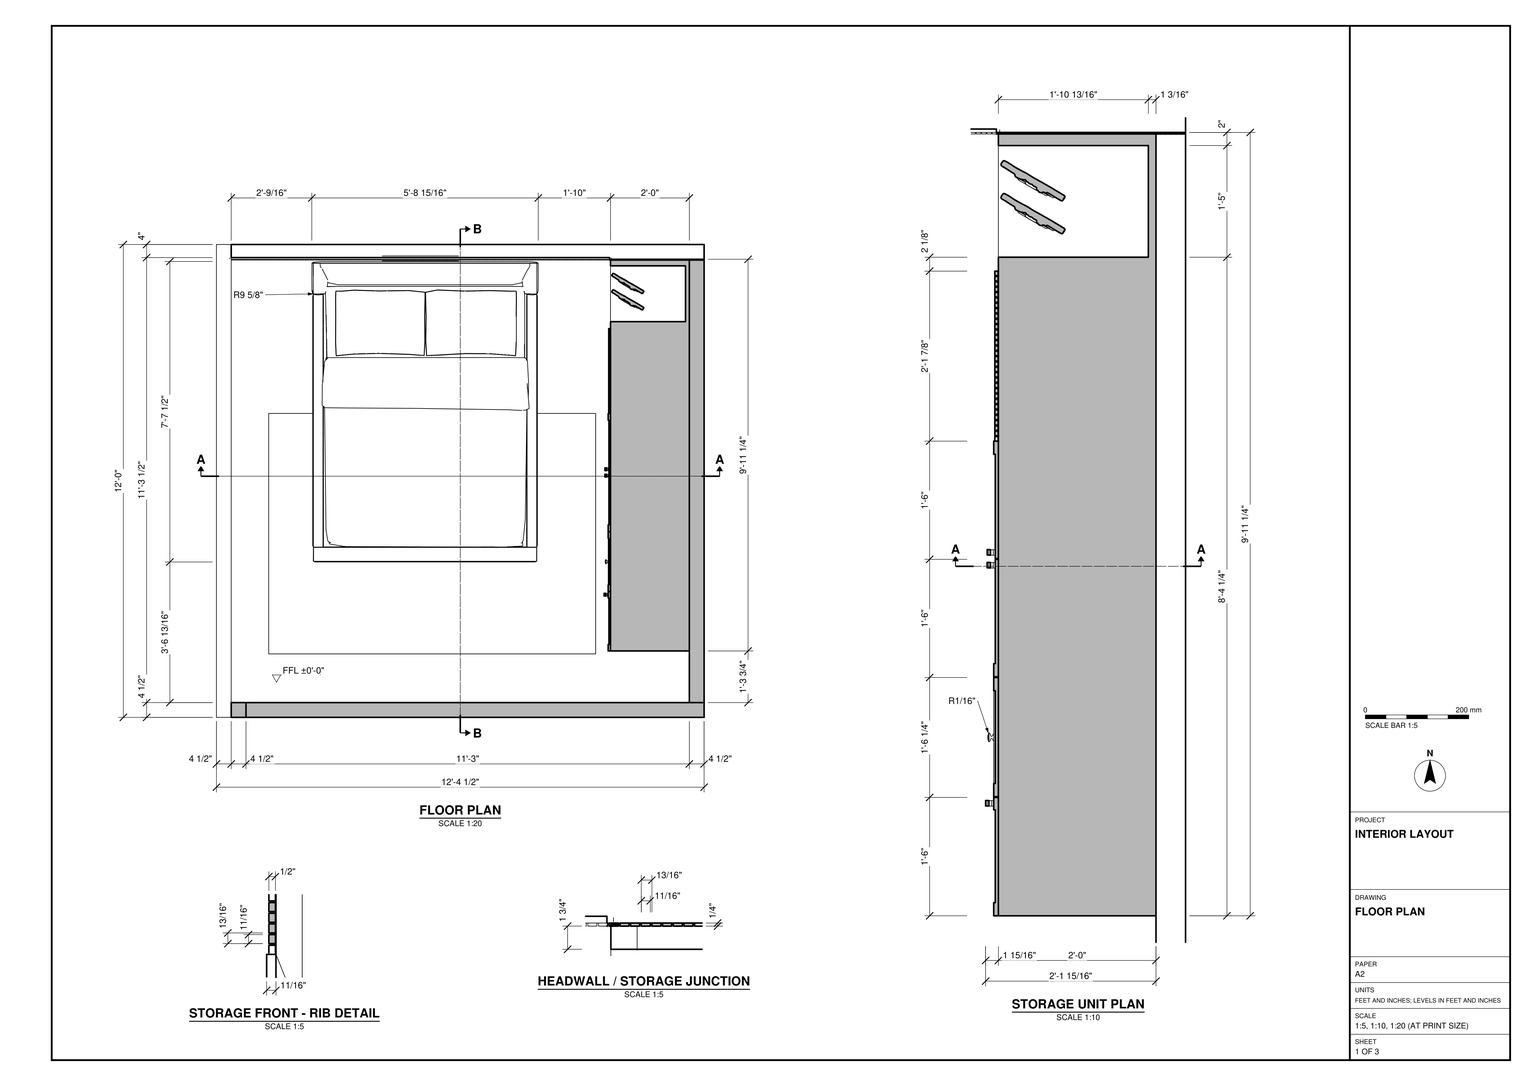
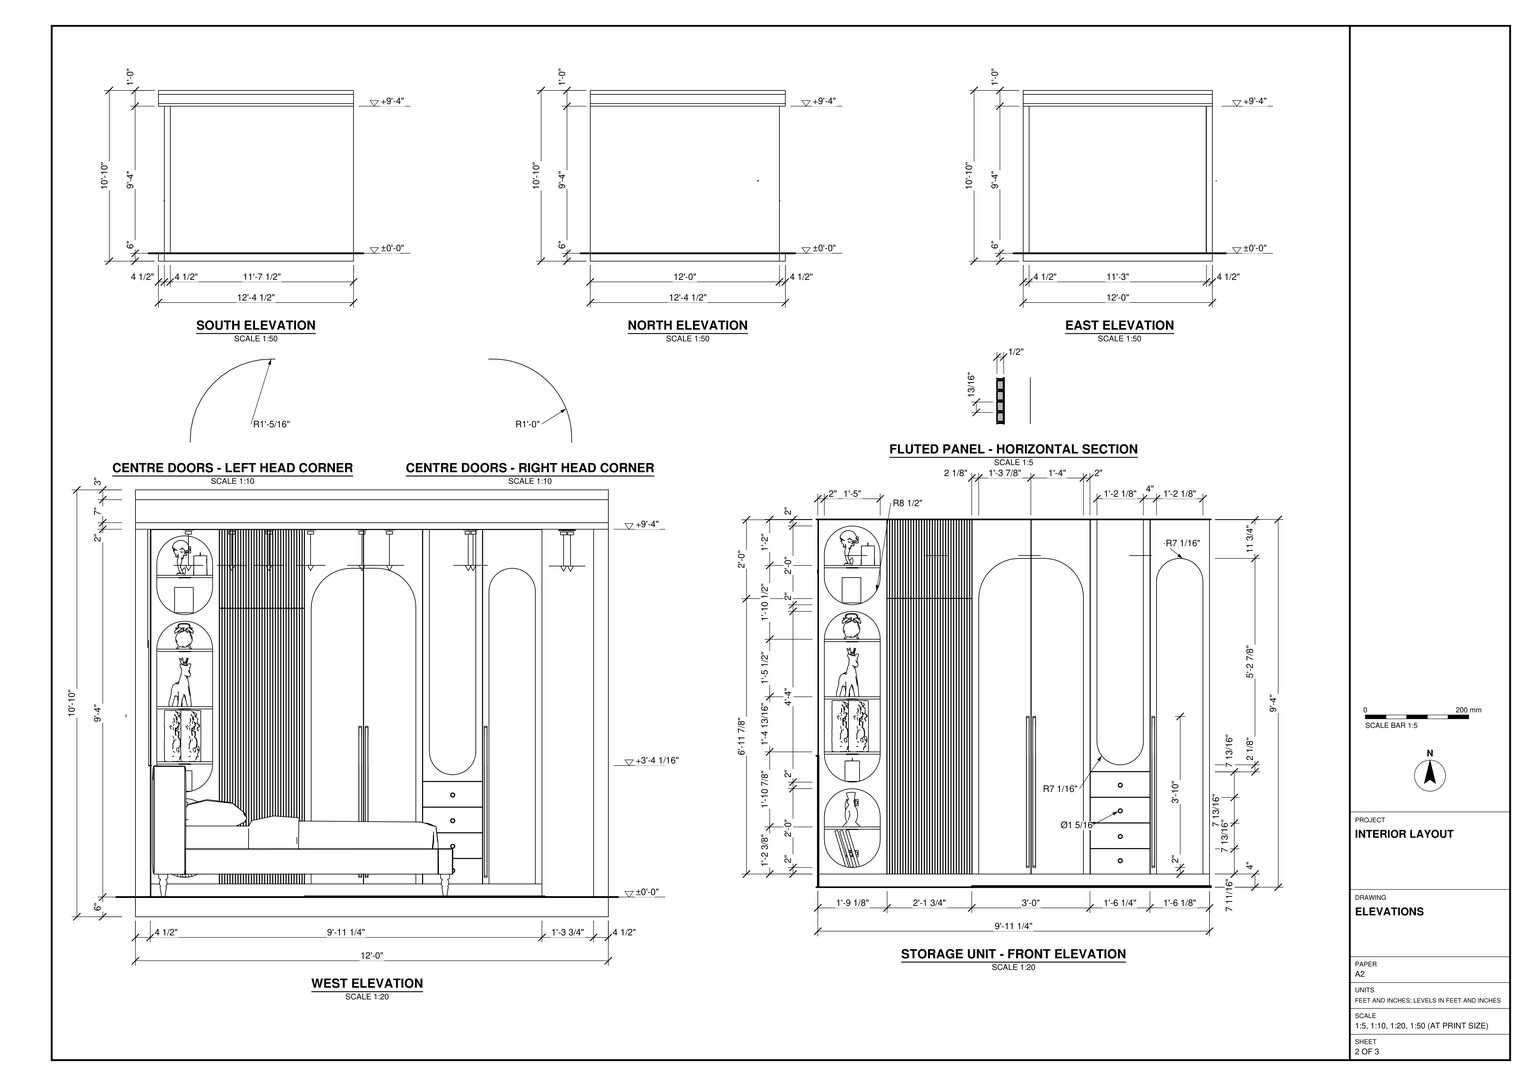
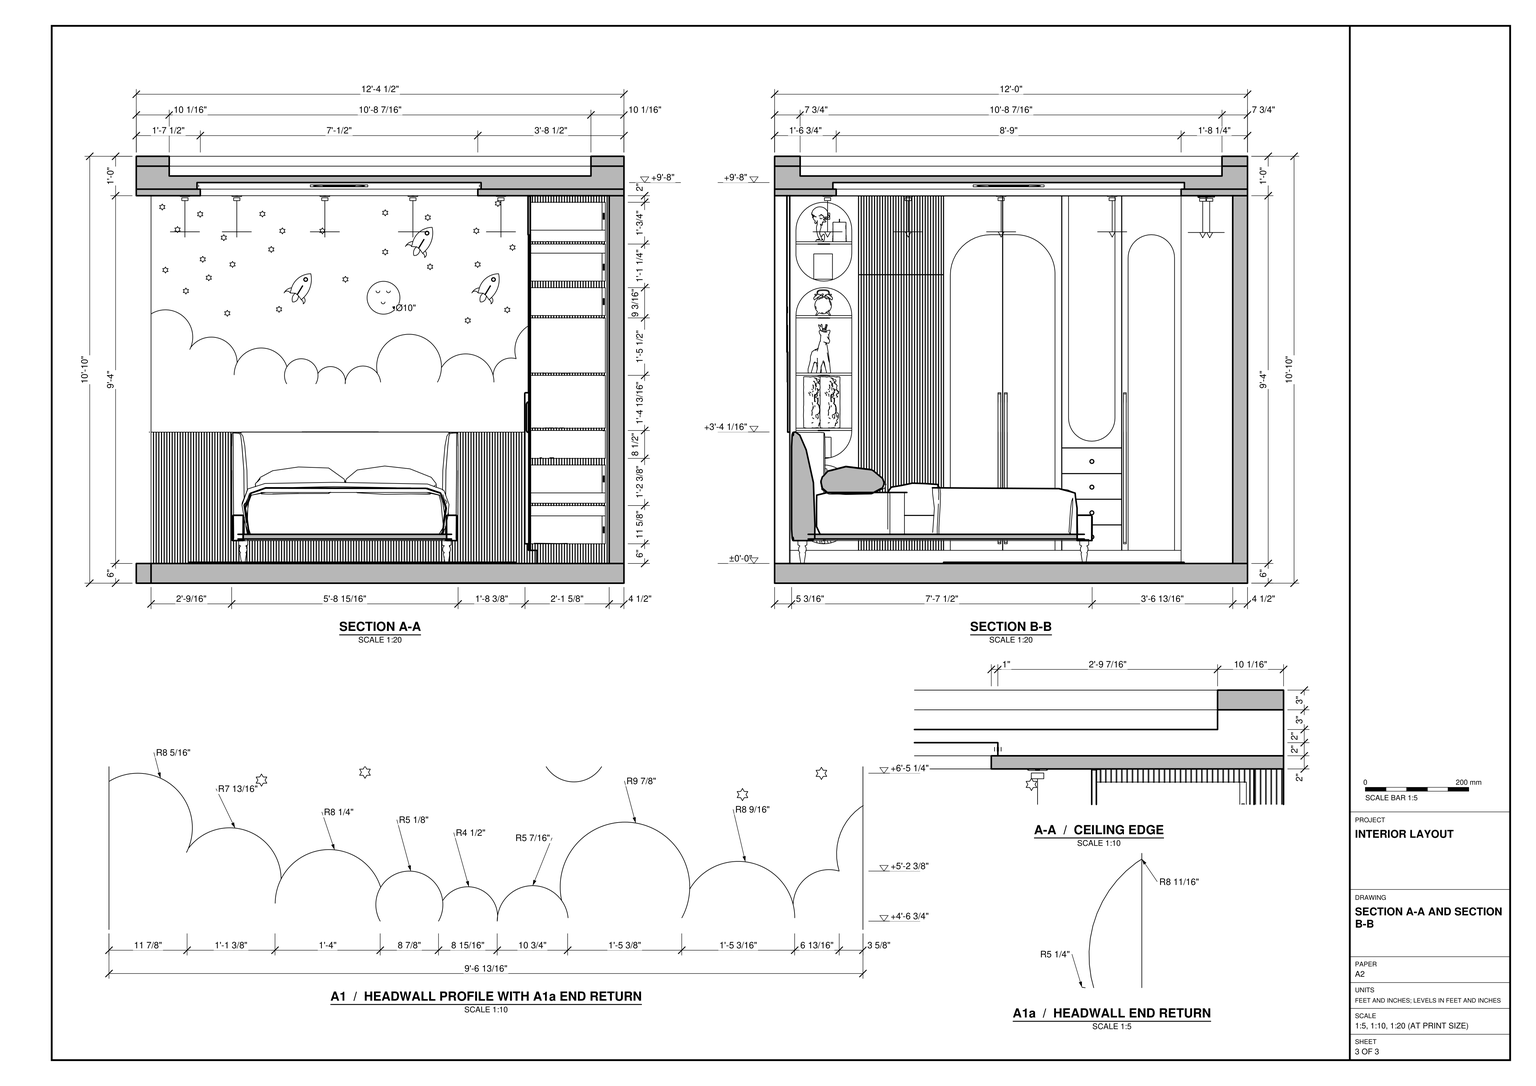
Build the bedroom interior in SketchUp from task_files/diagram_01.pdf. Work in feet and inches. Set the finished floor at ±0'-0" and make the overall model 12'-4 1/2" along X, 12'-2 7/8" along Y and 10'-10" high. Use the floor plan for placement and the sections for the floor slab, wall thicknesses and returns, clear height and stepped ceiling edge.

Place the bed with its head against the north wall and its foot facing the open floor area. Match the bed frame, raised headboard and footprint in plan and section. Behind the bed, model the ribbed lower panel and the scalloped headwall profile, including its curved end return. Fit the storage unit along the east wall with its fronts facing the bed. Follow the front elevation for the sequence of rounded display openings with shelves, a fluted bay, paired centre doors, a drawer stack and a tall end door. Use the enlarged details for the ribs and the junction with the headwall.

Decor and loose items, including the rug, shelf objects, wall decorations and lights, may be any suitable library components placed as shown. Keep the shell elements and each furniture or joinery piece in separate groups or components, and use components for repeated parts. Save one SketchUp model as output_files/bedroom_with_a_scalloped_headwall_and_fitted_storage.skp.

# SketchUp Ruby script. Lengths in inches.
U = 1.inch
M = Sketchup.active_model
def pt(a) = Geom::Point3d.new(a.map { |v| v * U })
def face(e, loops, mat)
  f = e.add_face(loops[0].map { |a| pt(a) })
  loops[1..].each { |l| e.add_face(l.map { |a| pt(a) }).erase! }
  f.material = f.back_material = mat if mat
  f
end
# faces: each face lists its corners as indices into pts; further lists are holes
def faces(e, pts, list, mat = nil) = list.each { |f| face(e, (f[0].is_a?(Array) ? f : [f]).map { |l| l.map { |i| pts[i] } }, mat) }
# xy, xz, yz: faces in a plane at the given z, y or x. An outline is a flat list of corners, or four numbers for a rectangle; further outlines are holes
def ring(l) = l.size == 4 ? [[l[0], l[1]], [l[2], l[1]], [l[2], l[3]], [l[0], l[3]]] : l.each_slice(2).to_a
def flat(e, list, mat, &to3) = list.each { |f| face(e, (f[0].is_a?(Array) ? f : [f]).map { |l| ring(l).map { |u, v| to3.(u, v) } }, mat) }
def xy(e, z, list, mat = nil) = flat(e, list, mat) { |x, y| [x, y, z] }
def xz(e, y, list, mat = nil) = flat(e, list, mat) { |x, z| [x, y, z] }
def yz(e, x, list, mat = nil) = flat(e, list, mat) { |y, z| [x, y, z] }
def lines(e, pts, list) = list.each { |a, b| e.add_line(pt(pts[a]), pt(pts[b])) }
# prism: a flat outline (further loops are holes) pulled along v
def prism(e, loops, v, mat = nil)
  f = face(e, loops, mat); d = Geom::Vector3d.new(v.map { |x| x * U })
  f.pushpull(f.normal.samedirection?(d) ? d.length : -d.length)
end
def box(e, o, s, mat = nil) = prism(e, [[o, [o[0] + s[0], o[1], o[2]], [o[0] + s[0], o[1] + s[1], o[2]], [o[0], o[1] + s[1], o[2]]]], [0, 0, s[2]], mat)
def at(x, y, z, deg = 0) = Geom::Transformation.translation(pt([x, y, z])) * Geom::Transformation.rotation(ORIGIN, Z_AXIS, deg.degrees)
def axes(o, x, y, z) = Geom::Transformation.new([*x, 0, *y, 0, *z, 0, *pt(o).to_a, 1])
def part(name) = M.definitions.add(name)
# library, detail: a bought-in or finely detailed component or shape, given as its bounding box
def library(name, o, s) = part(name).tap { |d| box(d.entities, o, s) }
def detail(e, o, s) = box(e.add_group.entities, o, s)
def put(e, d, t, mat = nil) = e.add_instance(d, t).tap { |i| i.material = mat if mat }
def group(e, t, mat = nil) = e.add_group.tap { |g| g.transformation = t; g.material = mat if mat }.entities
root = M.entities
M.materials.add("A08_Garnet_Shadow5").color = [28, 26, 30]
M.materials.add("DDR840RVS01100X").color = [126, 127, 125]
M.materials.add("Uniboard-L19-Putty-4K").color = [187, 181, 160]
c1 = part("Component\#11")
prism(c1.entities,[[[0.1875,0.74,0.15],[0.1875,0.74,16.59],[0.1875,0.74,16.61],[0.1875,0.73,16.625],[0.1875,0.73,16.64],[0.1875,0.72,16.66],[0.1875,0.71,16.67],[0.1875,0.7,16.68],[0.1875,0.6875,16.69],[0.1875,0.67,16.7],[0.1875,0.66,16.71],[0.1875,0.64,16.72],[0.1875,0.625,16.72],[0.1875,0.61,16.72],[0.18,0,16.72],[0.18,0,15.68],[0.18,0.14,15.68],[0.18,0.18,15.68],[0.18,0.22,15.67],[0.18,0.25,15.66],[0.18,0.29,15.64],[0.18,0.32,15.62],[0.18,0.35,15.59],[0.19,0.375,15.57],[0.1875,0.4,15.53],[0.1875,0.41,15.5],[0.1875,0.43,15.46],[0.1875,0.43,15.42],[0.1875,0.44,15.39],[0.1875,0.44,12.6],[0.1875,0.43,12.57],[0.1875,0.43,12.54],[0.1875,0.42,12.51],[0.1875,0.4,12.48],[0.19,0.38,12.45],[0.19,0.36,12.42],[0.18,0.34,12.4],[0.18,0.31,12.38],[0.18,0.28,12.37],[0.18,0.25,12.36],[0.18,0.22,12.35],[0.18,0.18,12.35],[0.18,0,12.35],[0.18,0,0],[0.1875,0.59,0],[0.1875,0.61,0],[0.1875,0.625,0.01],[0.1875,0.65,0.01],[0.1875,0.66,0.02],[0.1875,0.68,0.03],[0.1875,0.69,0.04],[0.1875,0.71,0.06],[0.1875,0.72,0.07],[0.1875,0.73,0.09],[0.1875,0.73,0.11],[0.1875,0.74,0.13]]],[-0.18,0,0],"A08_Garnet_Shadow5")
c2 = library("Interior Props 221 025",[-7.35,-1.5,-10.4],[14.7,1.56,20.81])
c3 = library("Decorative Deer 209 004",[-1.58,-4.16,0],[3.36,7.25,10.63])
c4 = library("Alarm Clock 114 007",[-2.86,-1.17,0.01],[5.71,2.99,7.86])
c5 = library("Interior Props 221 030",[-2.57,-3.63,-0.04],[5.13,7.27,11.89])
c6 = library("Decoration 111 063",[-2.51,-1.28,-0.03],[5.02,2.53,10.66])
c7 = library("Candle 111 040",[-2.11,-2.13,-0.02],[4.23,4.26,6.92])
c8 = library("Block 237 020",[-7.27,-8.35,0],[14.55,16.7,1.34])
c9 = part("Picture 288 039")
xz(c9.entities,-0.24,[[0.99,-15.21,-10.86,-15.18,-0.62,1.61],[0.99,-15.21,-0.62,1.61,10.87,-15.17],[0.67,-15.2,-0.25,2.42,-10.86,-15.16],[0.67,-15.2,10.89,1.32,-0.25,2.42],[0.67,-15.2,10.89,-15.1875,10.89,1.32],
  [-10.86,-15.18,-10.9,-1.29,-0.62,1.61],[10.87,-15.17,-0.62,1.61,10.9,-0.22],[-10.86,-15.16,-0.25,2.42,-10.89,2.08],[-10.9,-1.29,-10.9,15.22,-0.62,1.61],[10.9,-0.22,-0.62,1.61,10.88,15.2],
  [10.89,1.32,-1.31,15.2,-0.25,2.42],[10.89,1.32,10.89,15.21,-1.31,15.2],[-0.62,1.61,-10.9,15.22,-1.1,15.21],[-0.62,1.61,-1.1,15.21,10.88,15.2],[-10.89,2.08,-1.31,15.2,-10.9,15.2],
  [-10.89,2.08,-0.25,2.42,-1.31,15.2]])
xz(c9.entities,0,[[-12.08,-16.4,-12.1875,16.41,-11.52,3.74],[-12.08,-16.4,-11.45,-15.77,1.62,-15.8],[-12.08,-16.4,-11.52,3.74,-11.45,-15.77],[-12.08,-16.4,1.62,-15.8,11.44,-15.79],[-12.08,-16.4,11.44,-15.79,12.07,-16.375],
  [12.07,-16.375,11.44,-15.79,11.52,1.58],[12.07,-16.375,11.52,1.58,12.12,-2.15],[12.12,-2.15,11.52,1.58,12.07,16.36],[11.52,1.58,11.45,15.77,12.07,16.36],[-11.52,3.74,-12.1875,16.41,-11.43,15.75],
  [-11.43,15.75,-12.1875,16.41,-0.49,15.82],[11.45,15.77,-0.49,15.82,12.07,16.36],[-0.49,15.82,-12.1875,16.41,12.07,16.36]])
p = [[-12.19,-0.11,-1.23],[-12.2,-0.1,-16.51],[-11.65,-0.48,-4.41],[-11.48,-0.48,-15.9],[11.63,-0.48,-15.94],[12.2,-0.1,-16.52],
  [12.19,-0.11,-0.02],[-12.08,0,-16.4],[-12.12,-0.05,-16.53],[-12.21,-0.02,-16.4375],[-12.22,-0.0625,-3.89],[1.85,-0.0625,-16.53],
  [-0.625,-0.01,-16.52],[12.14,-0.02,-16.53],[12.21,-0.02,-16.43],[12.22,-0.0625,2.37],[12.07,0,-16.375],[-12.21,-0.01,0.01],
  [12.21,-0.01,16.52],[-12.1875,0,16.41],[12.12,0,-2.15],[-11.46,-0.47,-0.79],[-10.86,-0.24,-15.16],[-0.9,-0.47,-15.76],
  [0.67,-0.24,-15.2],[10.89,-0.24,-15.1875],[11.46,-0.47,1.83],[11.42,-0.47,15.71],[11.65,-0.48,15.96],[-11.45,0,-15.77],
  [-11.52,0,3.74],[-10.9,-0.24,-1.29],[-10.86,-0.24,-15.18],[1.62,0,-15.8],[0.99,-0.24,-15.21],[10.87,-0.24,-15.17],
  [11.44,0,-15.79],[10.9,-0.24,-0.22],[11.52,0,1.58],[-10.89,-0.24,2.08],[10.89,-0.24,1.32],[-12.2,-0.1,16.51],
  [-11.51,-0.48,15.89],[-12.22,-0.07,16.47],[12.07,0,16.36],[-10.9,-0.24,15.22],[-10.9,-0.24,15.2],[10.88,-0.24,15.2],
  [12.2,-0.1,16.51],[10.89,-0.24,15.21],[11.45,0,15.77],[12.22,-0.0625,16.53],[-11.43,0,15.75],[-1.71,-0.47,15.76],
  [-1.31,-0.24,15.2],[-0.49,0,15.82],[-1.1,-0.24,15.21],[-12.08,-0.01,16.52],[-1.82,-0.0625,16.53]]
faces(c9.entities,p,[[0,1,2],[1,3,2],[3,1,4],[1,5,4],[4,5,6],[7,8,9],[9,8,1],[1,0,10],
  [10,9,1],[8,11,1],[1,11,5],[8,7,12],[8,12,11],[12,13,11],[11,13,5],[5,13,14],
  [15,5,14],[6,5,15],[12,7,16],[16,13,12],[14,13,16],[17,9,10],[15,14,18],[7,9,17],
  [7,17,19],[20,18,14],[14,16,20],[2,3,21],[21,3,22],[3,4,23],[22,3,23],[24,23,4],
  [4,25,24],[25,4,26],[27,26,4],[27,4,28],[28,4,6],[23,24,22],[29,30,31],[31,32,29],
  [33,29,32],[32,34,33],[33,34,35],[35,36,33],[37,38,36],[36,35,37],[22,39,21],[26,40,25],
  [0,2,41],[41,2,42],[42,2,21],[17,10,43],[43,10,0],[18,20,44],[45,31,30],[43,0,41],
  [21,39,46],[42,21,46],[38,37,47],[28,6,48],[19,17,43],[48,6,15],[49,40,26],[47,50,38],
  [26,27,49],[51,15,18],[48,15,51],[30,52,45],[53,42,46],[46,54,53],[54,49,53],[53,49,27],
  [55,45,52],[56,45,55],[47,56,55],[50,47,55],[53,27,28],[42,53,28],[48,41,42],[42,28,48],
  [19,43,57],[18,19,57],[18,44,19],[57,43,41],[58,57,41],[48,58,41],[58,18,57],[51,18,58],
  [51,58,48]])
c10 = part("Candle 296 011")
p = [[-2.87,2.73,0.12],[-2.78,2.77,-0.01],[-2.85,-2.87,0.08],[-2.75,-2.73,-0.02],[2.76,-2.85,-0.01],[-0.35,-2.88,6.3],
  [2.73,-2.87,7.97],[2.875,-2.78,0.22],[-0.79,0,-0.03],[2.77,2.85,0.01],[2.87,2.73,0.11],[-2.74,2.86,0.08],
  [2.77,2.87,7.94],[0.21,2.875,0.13],[2.22,2.88,5.89],[-2.88,0.97,0.3],[-2.88,0.32,4.27],[-2.86,-2.77,4],
  [-2.84,-2.84,7.99],[2.88,0.02,5.47],[-2.88,-0.27,7.76],[-2.85,2.8,8],[2.86,2.75,7.99],[-2.73,2.87,7.95],
  [0.41,2.88,5.45],[2.86,-2.74,8.02],[-0.19,-1.07,7.78],[-1.39,-1.46,7.96],[0.21,-2.22,8.09],[0.71,-0.875,7.79],
  [1.92,-2.1,8.08],[1.55,-1.21,7.96],[-0.91,0.03,7.76],[-1.65,1.12,7.98],[-2.03,-1.45,8.07],[1.02,0.07,7.77],
  [2.04,-0.06,8.07],[-0.29,0.17,7.76],[-0.21,-0.06,7.76],[-0.21,0.07,8.34],[-0.11,0.04,7.78],[0.11,-0.07,9.22],
  [0.29,-0.01,9.13],[1.5,1.28,7.95],[-1.18,1.37,7.92],[0.16,1.13,7.79],[0.31,2.14,8.09],[-2.76,2.66,8.09],
  [2.75,2.76,8.07],[-2.75,-2.76,8.0625],[-2.21,0.78,8.09],[2.13,2.1,8.09]]
faces(c10.entities,p,[[0,1,2],[1,3,2],[3,4,2],[5,2,4],[5,4,6],[6,4,7],[3,8,4],[8,9,4],
  [4,9,10],[7,4,10],[3,1,8],[1,9,8],[0,11,1],[10,9,12],[13,1,11],[9,1,13],
  [14,9,13],[12,9,14],[15,0,2],[16,15,2],[16,2,17],[17,2,18],[18,2,5],[19,7,10],
  [0,16,20],[21,0,20],[19,10,22],[0,15,16],[11,0,21],[10,12,22],[23,11,21],[13,11,23],
  [24,13,23],[14,13,24],[6,7,25],[25,7,19],[16,17,20],[20,17,18],[25,19,22],[12,24,23],
  [14,24,12],[18,5,6],[20,18,21],[26,27,28],[28,29,26],[30,29,28],[30,31,29],[32,33,34],
  [32,34,27],[26,32,27],[35,29,31],[36,35,31],[26,37,32],[38,37,26],[26,35,38],[29,35,26],
  [38,39,37],[35,40,38],[41,39,38],[41,38,40],[41,40,42],[36,43,35],[32,44,33],[32,45,44],
  [45,32,37],[40,37,39],[37,40,35],[39,42,40],[35,45,37],[43,45,35],[46,44,45],[43,46,45],
  [44,46,33],[23,21,47],[48,23,47],[12,23,48],[22,12,48],[6,49,18],[25,49,6],[47,21,49],
  [21,18,49],[25,30,49],[25,48,30],[25,22,48],[28,27,34],[31,30,36],[34,33,50],[36,51,43],
  [33,47,50],[46,47,33],[43,51,46],[50,47,49],[34,50,49],[28,34,49],[30,28,49],[30,48,36],
  [48,51,36],[46,48,47],[51,48,46],[42,39,41]])
c11 = library("Crowd Pleaser Bed",[-34.48,-45.67,0],[68.96,91.51,40.05])
c12 = part("Carpet v15 (4)")
xy(c12.entities,0,[[-70.87,0,47.24,78.74]])
xy(c12.entities,0.39,[[-70.87,0,47.24,78.74]],"DDR840RVS01100X")
xz(c12.entities,0,[[-70.87,0,47.24,0.39]])
xz(c12.entities,78.74,[[-70.87,0,47.24,0.39]])
yz(c12.entities,-70.87,[[0,0,78.74,0.39]])
yz(c12.entities,47.24,[[0,0,78.74,0.39]])
c13 = library("Group\#4",[-1.63,0,0],[25.63,119.28,112])
c14 = library("Group\#2",[-0.5,-0.5,0],[144.5,5,112])
c15 = library("Group\#12",[0,0,0],[148.5,144,12])
c16 = library("Group\#17",[0,0,0],[8.9,8.9,12.62])
xz(root,146.875,[[20.87,60.82,20.98,61.01,21.19,61.01,21.09,61.19,21.19,61.38,20.98,61.38,20.87,61.57,20.76,61.38,20.54,61.38,20.65,61.19,20.76,61.01],[20.54,61.01,20.76,61.01,20.65,61.19]])
put(root,c1,axes([119.53,75.12,12],[0,4.59482,0],[-1.67085,0,0],[0,0,2.75092]))
put(root,c1,axes([119.53,73.17,12],[0,4.59482,0],[-1.67085,0,0],[0,0,2.75092]))
put(root,c1,axes([119.29,36.91,12],[0,4.59482,0],[-1.67085,0,0],[0,0,2.75092]))
put(root,c2,axes([125.52,127.54,55.07],[0.64952,-0.375,0],[0.5,0.86603,0],[0,0,0.75573]))
put(root,c2,axes([125.52,132.54,55.07],[0.64952,-0.375,0],[0.5,0.86603,0],[0,0,0.75573]))
put(root,c3,axes([127.15,130.29,63.88],[0.6048,-1.2737,0],[1.2737,0.6048,0],[0,0,1.41]))
put(root,c4,at(123.72,129.23,81.5,-90))
put(root,c5,axes([126.47,129.43,24.35],[0.34857,-0.93728,0],[0.93728,0.34857,0],[0,0,0.89]))
put(root,c6,at(124.81,130.23,103.98,-90))
put(root,c7,at(124.94,124.25,103.98,-90))
put(root,c8,axes([126.83,131.78,17.8125],[0.7,0,0],[0,-0.20264,-0.67003],[0,0.67003,-0.20264]))
put(root,c8,axes([126.83,130.32,17.8125],[0.7,0,0],[0,-0.20264,-0.67003],[0,0.67003,-0.20264]))
put(root,c8,axes([126.22,128.49,17.89],[0.7,0,0],[0,-0.20264,-0.67003],[0,0.67003,-0.20264]))
put(root,c9,axes([123.55,129.23,96.43],[0,-0.23328,0],[0.23328,0,0],[0,0,0.23328]))
put(root,c10,axes([124.99,129.01,38.25],[0.77,0,0],[0,0.77,0],[0,0,0.77]))
put(root,c11,at(63.52,92.99,6))
put(root,c12,axes([75.65,19.32,6],[0.84295,0,0],[0,0.93,0],[0,0,0.93]))
g1 = group(root,at(4.5,0,0))
xy(g1,0,[[-4.5,0,0,144],[0,0,144,144]])
xy(g1,6,[[-4.5,0,0,144],[0,0,144,144]])
xz(g1,0,[[-4.5,0,0,6],[0,0,144,6]])
xz(g1,144,[[-4.5,0,0,6],[0,0,144,6]])
yz(g1,-4.5,[[0,0,144,6]])
yz(g1,0,[[0,0,144,6]])
yz(g1,144,[[0,0,144,6]])
g2 = group(root,at(144,4.5,6))
box(g2,[0,0,0],[4.5,135,112])
g3 = group(root,at(9,0,6))
box(g3,[0,0,0],[139.5,4.5,112])
put(root,c13,at(120,20.22,6),"Uniboard-L19-Putty-4K")
put(root,c14,at(4.5,139.5,6))
g4 = group(root,at(4.5,0,6))
box(g4,[0,0,0],[144,4.5,112])
put(root,c15,at(0,0,118))
put(root,c16,at(106.59,123.42,105.38))
put(root,c16,at(106.59,98.88,105.38))
put(root,c16,at(106.59,70.57,105.38))
put(root,c16,at(106.59,36.76,105.38))
put(root,c16,at(79.78,123.42,105.38))
put(root,c16,at(52.97,123.42,105.38))
put(root,c16,at(26.16,123.42,105.38))
put(root,c16,at(10.36,110.22,105.38))
put(root,c16,at(10.36,86.22,105.38))
put(root,c16,at(10.36,62.22,105.38))
put(root,c16,at(10.36,38.22,105.38))
put(root,c16,at(22.18,9.19,105.17))
put(root,c16,at(46.18,9.19,105.17))
put(root,c16,at(70.18,9.19,105.17))
put(root,c16,at(94.18,9.19,105.17))
put(root,c16,at(127.74,7.07,105.17))
g5 = group(root,at(0,0,6))
xy(g5,0,[[0,0,4.5,144]])
